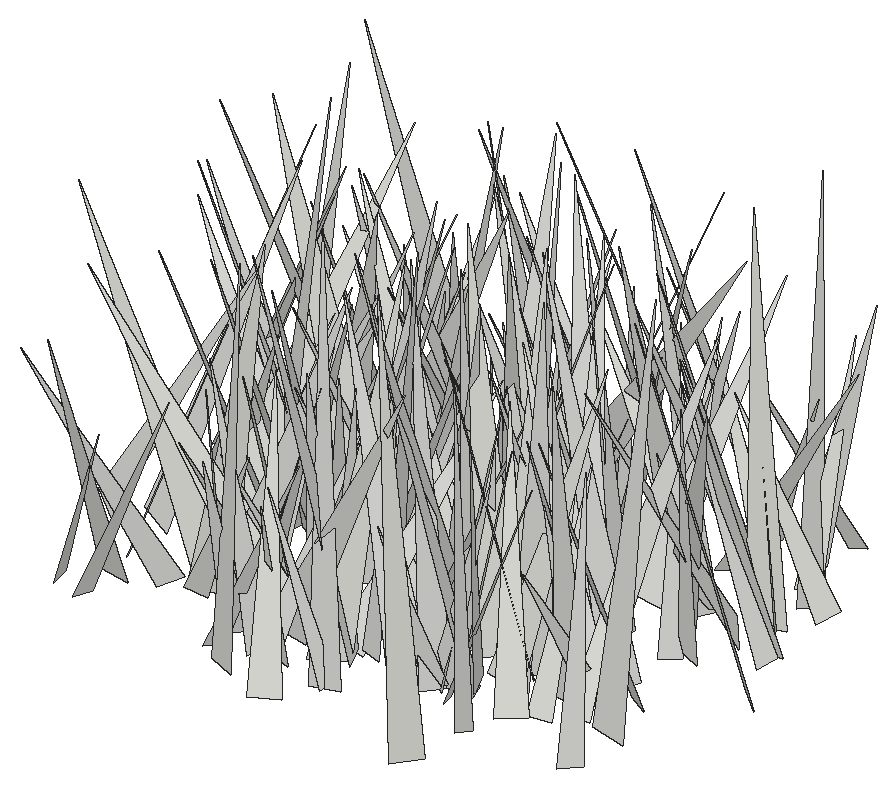
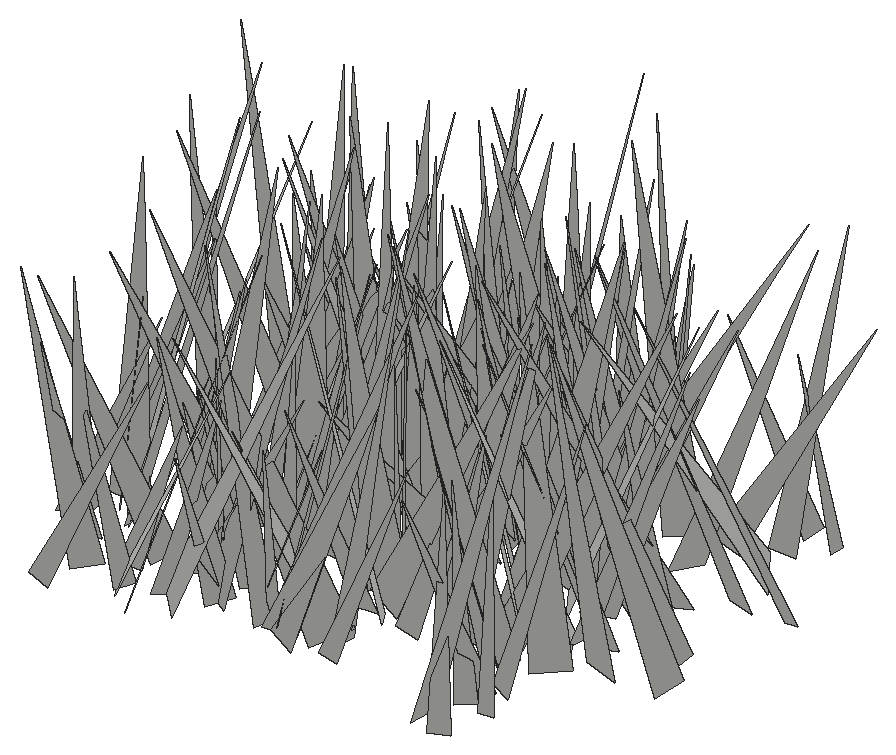
# SketchUp Ruby script. Lengths in inches.
U = 1.inch
M = Sketchup.active_model
def pt(a) = Geom::Point3d.new(a.map { |v| v * U })
def face(e, loops, mat)
  f = e.add_face(loops[0].map { |a| pt(a) })
  loops[1..].each { |l| e.add_face(l.map { |a| pt(a) }).erase! }
  f.material = f.back_material = mat if mat
  f
end
# faces: each face lists its corners as indices into pts; further lists are holes
def faces(e, pts, list, mat = nil) = list.each { |f| face(e, (f[0].is_a?(Array) ? f : [f]).map { |l| l.map { |i| pts[i] } }, mat) }
# xy, xz, yz: faces in a plane at the given z, y or x. An outline is a flat list of corners, or four numbers for a rectangle; further outlines are holes
def ring(l) = l.size == 4 ? [[l[0], l[1]], [l[2], l[1]], [l[2], l[3]], [l[0], l[3]]] : l.each_slice(2).to_a
def flat(e, list, mat, &to3) = list.each { |f| face(e, (f[0].is_a?(Array) ? f : [f]).map { |l| ring(l).map { |u, v| to3.(u, v) } }, mat) }
def xy(e, z, list, mat = nil) = flat(e, list, mat) { |x, y| [x, y, z] }
def xz(e, y, list, mat = nil) = flat(e, list, mat) { |x, z| [x, y, z] }
def yz(e, x, list, mat = nil) = flat(e, list, mat) { |y, z| [x, y, z] }
def lines(e, pts, list) = list.each { |a, b| e.add_line(pt(pts[a]), pt(pts[b])) }
# prism: a flat outline (further loops are holes) pulled along v
def prism(e, loops, v, mat = nil)
  f = face(e, loops, mat); d = Geom::Vector3d.new(v.map { |x| x * U })
  f.pushpull(f.normal.samedirection?(d) ? d.length : -d.length)
end
def box(e, o, s, mat = nil) = prism(e, [[o, [o[0] + s[0], o[1], o[2]], [o[0] + s[0], o[1] + s[1], o[2]], [o[0], o[1] + s[1], o[2]]]], [0, 0, s[2]], mat)
def at(x, y, z, deg = 0) = Geom::Transformation.translation(pt([x, y, z])) * Geom::Transformation.rotation(ORIGIN, Z_AXIS, deg.degrees)
def axes(o, x, y, z) = Geom::Transformation.new([*x, 0, *y, 0, *z, 0, *pt(o).to_a, 1])
def part(name) = M.definitions.add(name)
# library, detail: a bought-in or finely detailed component or shape, given as its bounding box
def library(name, o, s) = part(name).tap { |d| box(d.entities, o, s) }
def detail(e, o, s) = box(e.add_group.entities, o, s)
def put(e, d, t, mat = nil) = e.add_instance(d, t).tap { |i| i.material = mat if mat }
def group(e, t, mat = nil) = e.add_group.tap { |g| g.transformation = t; g.material = mat if mat }.entities
root = M.entities
c1 = part("fur_instance\#9")
p = [[0.8125,0,1.79],[0.67,-0.02,1.48],[0,-0.11,0],[0,0.11,0]]
faces(c1.entities,p,[[0,1,2,3]])
put(root,c1,axes([98,397.39,-27.1],[-0.65259,-3.58567,0.77528],[-3.62638,0.74954,0.41412],[0.55447,0.682,3.62097]))
put(root,c1,axes([89.63,398.5625,-27.1],[-0.57876,-6.04691,0.53315],[-6.05695,0.61084,0.35302],[0.40347,0.49606,6.06428]))
put(root,c1,axes([99.22,394.98,-27.1],[-1.93628,5.55,0.46539],[5.55779,1.89356,0.54185],[-0.36056,-0.61659,5.85304]))
put(root,c1,axes([96.62,395.82,-27.1],[3.17531,6.56755,2.54139],[6.79761,-3.58673,0.77578],[-1.83954,-1.91744,7.25351]))
put(root,c1,axes([95.52,398.04,-27.1],[2.55514,-3.36467,0.69917],[-3.31318,-2.64324,-0.61213],[-0.91251,0.1757,4.18031]))
put(root,c1,axes([100.41,397.04,-27.1],[-3.8674,0.14725,0.40736],[0.1724,3.88071,0.23399],[0.39736,-0.25058,3.86312]))
put(root,c1,axes([105.92,394.58,-27.1],[-8.22184,1.12863,0.67504],[0.91948,7.98903,-2.15825],[0.94024,2.05661,8.01339]))
put(root,c1,axes([88.22,397.28,-27.1],[3.62066,0.28745,0.41277],[0.34104,-3.60783,-0.479],[-0.36973,-0.51296,3.60033]))
put(root,c1,axes([95.45,396.87,-27.1],[4.11337,-1.35782,0.42666],[-1.42017,-4.00175,0.95638],[-0.09392,1.04301,4.22479]))
put(root,c1,axes([95.85,397.16,-27.1],[-3.35833,-3.2337,1.73378],[-3.57177,3.41915,-0.54142],[0.83981,1.61055,4.63056]))
put(root,c1,axes([89.6,396.83,-27.1],[4.44559,-0.41699,0.42413],[-0.48383,-4.39553,0.74982],[-0.34594,0.78895,4.4017]))
put(root,c1,axes([96.93,397.62,-27.1],[-5.40914,1.11965,1.3835],[1.23539,5.5484,0.3398],[1.28121,-0.62292,5.51334]))
put(root,c1,axes([91.48,399.41,-27.1],[0.83306,-5.07313,1.39633],[-4.3947,-1.44829,-2.63999],[-2.89363,0.73905,4.41148]))
put(root,c1,axes([103.39,399.39,-27.1],[1.75124,-3.26229,0.83742],[-3.12175,-1.92651,-0.97669],[-1.26432,0.23809,3.57148]))
put(root,c1,axes([96.93,399.07,-27.1],[2.93254,-6.52755,1.0505],[-6.19008,-2.30697,2.94501],[2.32281,2.09313,6.52193]))
put(root,c1,axes([96.53,399.75,-27.1],[-0.29394,-4.28793,0.2812],[-4.0742,0.18848,-1.38464],[-1.36614,0.36048,4.06885]))
put(root,c1,axes([96.73,400.14,-27.1],[-3.34858,-4.98605,1.16696],[-4.83329,3.53804,1.24784],[1.69169,0.23891,5.87509]))
put(root,c1,axes([99.67,399.53,-27.1],[-7.3935,-3.44968,1.78048],[-3.41196,7.60131,0.55924],[1.85173,0.23234,8.13949]))
put(root,c1,axes([96.3,399.9,-27.1],[-7.10232,2.48969,0.17848],[2.39972,6.66255,2.55443],[-0.68683,-2.46683,7.07929]))
put(root,c1,axes([92.61,399.39,-27.1],[1.69765,-3.69471,0.41656],[-3.54176,-1.46758,1.41724],[1.13153,0.9496,3.81108]))
put(root,c1,axes([100.46,396.83,-27.1],[1.13757,8.04859,1.54719],[7.76789,-1.55698,2.3882],[-2.61411,-1.12413,7.76984]))
put(root,c1,axes([97.34,397.36,-27.1],[-2.89965,3.32427,1.06428],[2.78447,3.03733,-1.90073],[2.1048,0.5615,3.98069]))
put(root,c1,axes([110.67,397.78,-27.1],[-4.9436,1.78617,0.77223],[1.56135,4.89918,-1.33648],[1.16143,1.01666,5.08364]))
put(root,c1,axes([106.16,397.46,-27.1],[-6.18556,-0.57175,1.0735],[-0.94708,5.75521,-2.39186],[0.76312,2.5082,5.73298]))
put(root,c1,axes([104.51,400.33,-27.1],[-4.3896,-2.50757,2.34029],[-2.3133,4.97071,0.98703],[2.5325,0.19407,4.95805]))
put(root,c1,axes([102.49,399.06,-27.1],[-6.29408,3.56033,1.19684],[3.6784,6.31519,0.55815],[0.76008,-1.07993,7.20971]))
put(root,c1,axes([103.33,399.73,-27.1],[0.04539,-4.24616,1.86431],[-4.44886,0.48634,1.21602],[1.30888,1.80033,4.06857]))
put(root,c1,axes([95.48,399.4,-27.1],[5.08569,0.11573,0.95874],[0.07501,-5.17107,0.22632],[-0.96278,0.20845,5.08197]))
put(root,c1,axes([93.01,399.72,-27.1],[-2.73382,6.12597,3.74599],[6.6709,3.64992,-1.10045],[2.6569,-2.86083,6.61742]))
put(root,c1,axes([96.35,401.17,-27.1],[-3.41179,-1.77285,0.16017],[-1.67154,3.30984,1.02951],[0.61205,-0.84317,3.70451]))
put(root,c1,axes([96.98,401.18,-27.1],[3.24454,-4.71501,1.03025],[-4.7617,-3.32972,-0.24278],[-0.78672,0.70811,5.71834]))
put(root,c1,axes([104.32,398.85,-27.1],[3.89284,1.77366,0.49192],[1.64576,-3.86945,0.92782],[-0.82421,0.65077,4.17603]))
put(root,c1,axes([104.79,399.78,-27.1],[-7.44301,-3.63877,0.95843],[-3.76282,7.20814,-1.85509],[0.01898,2.08796,8.0745]))
put(root,c1,axes([98.05,400.78,-27.1],[4.42383,-2.92058,1.2942],[-2.99041,-4.56361,-0.07677],[-1.12348,0.64702,5.30039]))
put(root,c1,axes([100.23,399.66,-27.1],[-1.46329,-3.87448,2.4887],[-4.52721,1.6881,-0.03379],[0.84239,2.34204,4.14146]))
put(root,c1,axes([108.59,402.04,-27.1],[2.63611,-2.6678,0.56163],[-2.26437,-2.5776,-1.61563],[-1.51829,-0.78771,3.38467]))
put(root,c1,axes([99.3,398.49,-27.1],[-5.55671,4.70477,2.20019],[4.40361,5.97611,-1.65743],[2.7539,-0.06297,7.08977]))
put(root,c1,axes([103.92,400.03,-27.1],[4.05853,2.67005,1.15678],[2.78357,-4.14094,-0.20805],[-0.84796,-0.81387,4.85361]))
put(root,c1,axes([107.83,401.4,-27.1],[0.14601,-6.62439,2.10053],[-6.94709,-0.08453,0.21629],[0.18059,2.1039,6.62247]))
put(root,c1,axes([106.84,399.27,-27.1],[-4.29612,3.71614,0.38084],[3.69784,4.31285,-0.36964],[0.52979,0.03157,5.66831]))
put(root,c1,axes([101.72,403.07,-27.1],[-1.16201,-7.65185,1.0654],[-7.72512,1.16361,-0.06847],[0.09162,1.06366,7.73928]))
put(root,c1,axes([91.57,401.52,-27.1],[-7.37091,1.53228,0.84327],[1.65266,7.29739,1.18581],[0.57246,-1.33774,7.43452]))
put(root,c1,axes([105.21,402.41,-27.1],[-4.80805,-4.95386,1.3489],[-5.02147,4.92244,0.17909],[1.0701,0.84054,6.90116]))
put(root,c1,axes([107.86,401.81,-27.1],[1.52237,-3.55739,1.37163],[-3.65271,-1.78416,-0.57315],[-1.09275,1.00785,3.82677]))
put(root,c1,axes([103.53,399.18,-27.1],[-7.58228,1.17889,0.51367],[1.00041,7.33787,-2.07353],[0.80796,1.97752,7.38791]))
put(root,c1,axes([103.68,399.24,-27.1],[3.73526,4.02595,0.93613],[3.5763,-3.78049,1.98866],[-2.07237,0.73241,5.11915]))
put(root,c1,axes([109.67,402.8125,-27.1],[-3.13069,-4.74867,0.6646],[-4.79451,3.11096,-0.35688],[0.06511,0.75154,5.67659]))
put(root,c1,axes([107.67,399.79,-27.1],[-0.4926,4.67354,0.05511],[4.67276,0.49124,0.10792],[-0.10156,-0.0661,4.69819]))
put(root,c1,axes([110.29,400.34,-27.1],[2.12447,7.8086,2.15105],[8.03257,-2.31646,0.47574],[-1.03873,-1.94278,8.07844]))
put(root,c1,axes([99.2,399.68,-27.1],[-0.72981,5.66267,0.18679],[5.27184,0.7477,-2.06932],[2.0757,0.09199,5.32132]))
put(root,c1,axes([95.5,403.39,-27.1],[-0.07367,-4.26522,0.50041],[-4.16979,0.19077,1.01214],[1.02732,0.46845,4.14405]))
put(root,c1,axes([105.45,402.17,-27.1],[1.282,-6.99581,3.06835],[-7.6361,-1.26107,0.31524],[-0.21483,3.07701,7.10532]))
put(root,c1,axes([105.08,401.09,-27.1],[0.03903,6.40601,1.64221],[6.43648,0.34027,-1.48032],[1.51842,-1.60705,6.23275]))
put(root,c1,axes([98.98,402.36,-27.1],[7.15031,1.42356,2.57616],[1.59453,-7.56218,-0.24693],[-2.47399,-0.75958,7.28646]))
put(root,c1,axes([108.72,400.625,-27.1],[-1.96871,3.37657,0.07437],[3.27614,1.93014,-0.90775],[0.82077,0.39482,3.80171]))
put(root,c1,axes([101.26,400.78,-27.1],[4.64309,0.99306,0.50279],[0.80416,-4.48393,1.43003],[-0.7696,1.30595,4.52764]))
put(root,c1,axes([100.41,402.65,-27.1],[-3.73947,1.85603,0.44676],[1.90802,3.6015,1.00834],[-0.06253,-1.10111,4.05114]))
put(root,c1,axes([96.15,403.49,-27.1],[4.14097,0.37336,0.37849],[0.46882,-3.96604,-1.21698],[-0.25072,-1.24957,3.97567]))
put(root,c1,axes([106.59,404.04,-27.1],[-1.84979,-4.95748,0.73449],[-4.97918,1.90688,0.3307],[0.56907,0.57009,5.281]))
put(root,c1,axes([95.66,403.45,-27.1],[0.8315,-3.67241,0.7269],[-3.73531,-0.86356,-0.09004],[-0.24991,0.6885,3.76429]))
put(root,c1,axes([95.33,404.04,-27.1],[0.2797,-5.08952,0.70223],[-5.01624,-0.11848,1.13926],[1.11073,0.74654,4.96825]))
put(root,c1,axes([108.11,402.18,-27.1],[-4.76226,4.46867,0.77555],[4.53262,4.64929,1.04363],[-0.16086,-1.29026,6.44663]))
put(root,c1,axes([93.45,403.39,-27.1],[-3.66042,-4.84933,0.70173],[-4.78346,3.34689,-1.82316],[-1.06154,1.63996,5.79575]))
put(root,c1,axes([102.76,402.32,-27.1],[-6.8831,0.44539,2.18741],[0.27023,7.20464,-0.61666],[2.21588,0.50489,6.86987]))
put(root,c1,axes([92.375,402.62,-27.1],[1.25839,-5.65908,2.69216],[-6.0262,-0.33916,2.10388],[1.71982,2.95233,5.40207]))
put(root,c1,axes([103.74,402.46,-27.1],[-6.05615,5.17907,2.30301],[5.46239,6.23254,0.34836],[1.51293,-1.77094,7.96105]))
put(root,c1,axes([102.32,403.3,-27.1],[2.05705,-3.40779,1.21765],[-3.60141,-2.06493,0.30505],[-0.3543,1.20424,3.9688]))
put(root,c1,axes([92.71,405.33,-27.1],[-2.90954,-6.16313,0.64564],[-6.10361,2.97343,0.8781],[1.07095,0.20243,6.75859]))
put(root,c1,axes([86.18,402.37,-27.1],[3.46284,5.45761,0.55951],[5.19477,-3.049,-2.40992],[1.76435,-1.73432,5.99742]))
put(root,c1,axes([98.26,405.3,-27.1],[-5.70608,-2.81682,0.48614],[-2.67601,5.6456,1.30244],[1.0049,-0.96065,6.22877]))
put(root,c1,axes([96.38,404.87,-27.1],[-4.22859,-0.79072,0.99748],[-0.41595,4.12901,1.5098],[1.20299,-1.35177,4.02824]))
put(root,c1,axes([94.06,405.22,-27.1],[-1.823,-5.96341,0.88128],[-5.94354,1.93183,0.77754],[1.00658,0.60664,6.18716]))
put(root,c1,axes([100.49,404.15,-27.1],[6.63287,-1.89646,1.66739],[-1.83678,-6.83922,-0.47211],[-1.73291,-0.0097,6.88248]))
put(root,c1,axes([105.97,400.49,-27.1],[-6.32088,1.55628,0.92222],[1.03646,5.86264,-2.78949],[1.48264,2.53644,5.88169]))
put(root,c1,axes([107.03,403.59,-27.1],[-1.92463,-5.23066,1.71698],[-5.26178,1.21283,-2.20335],[-1.6191,2.27625,5.1195]))
put(root,c1,axes([104.8125,402.0625,-27.1],[-1.18605,7.62635,1.82441],[7.84154,1.15487,0.27022],[0.00582,-1.84431,7.7133]))
put(root,c1,axes([93.46,402.88,-27.1],[0.89706,4.01856,0.51185],[4.05094,-0.89322,-0.08685],[-0.02607,-0.51851,4.11655]))
put(root,c1,axes([92.5,405.0625,-27.1],[6.03259,-1.06555,0.38284],[-1.02373,-6.01977,-0.62323],[-0.48366,-0.54868,6.09418]))
put(root,c1,axes([102.65,402.875,-27.1],[-4.5808,2.50643,0.71678],[2.42315,4.62824,-0.69815],[0.96142,0.27723,5.1748]))
put(root,c1,axes([88.34,402.5,-27.1],[3.15625,6.97995,0.87784],[7.00121,-3.02246,-1.14023],[0.68808,-1.26383,7.57506]))
put(root,c1,axes([112.61,405.41,-27.1],[-5.20648,-5.71637,1.32602],[-5.85189,5.18966,-0.6046],[0.43665,1.3904,7.70836]))
put(root,c1,axes([108.56,403.31,-27.1],[-7.87651,1.28049,0.44694],[1.23259,7.85729,-0.78901],[0.56579,0.70864,7.94081]))
put(root,c1,axes([89.11,399.98,-27.1],[6.66219,5.05954,0.23915],[4.47229,-6.06129,3.64695],[-2.37798,2.77537,7.52884]))
put(root,c1,axes([98.6875,404.67,-27.1],[-2.55012,3.64542,1.48438],[3.93085,2.44958,0.73729],[0.20222,-1.64502,4.38733]))
put(root,c1,axes([97.36,403.51,-27.1],[5.64038,0.84844,0.8162],[0.68974,-5.61874,1.07421],[-0.95409,0.95384,5.60177]))
put(root,c1,axes([96.61,403.33,-27.1],[6.53232,-2.04401,3.08815],[-2.89411,-6.72439,1.67109],[-2.31057,2.64395,6.63752]))
put(root,c1,axes([103.83,406.2,-27.1],[-3.87501,-4.05549,0.17386],[-4.05477,3.85598,-0.42797],[-0.18982,0.42113,5.59281]))
put(root,c1,axes([95.58,404.09,-27.1],[6.99973,1.86447,1.44835],[1.77883,-7.14461,0.6004],[-1.55233,0.22015,7.21886]))
put(root,c1,axes([89,405.9,-27.1],[3.52002,-2.83902,0.00242],[-2.82378,-3.50072,0.47096],[0.29379,0.3681,4.49764]))
put(root,c1,axes([106.98,403.66,-27.1],[0.16958,6.97336,1.46095],[6.91324,0.19239,-1.72074],[1.72314,-1.45812,6.75984]))
put(root,c1,axes([97.67,404.49,-27.1],[4.97353,-2.18793,2.98402],[-2.79783,-5.49524,0.634],[-2.42149,1.85546,5.39639]))
put(root,c1,axes([103.84,404.8125,-27.1],[-5.54027,1.19429,0.93196],[1.15956,5.61711,-0.30487],[0.97482,0.10593,5.65933]))
put(root,c1,axes([109.23,408.98,-27.1],[-5.37416,-4.85351,0.14678],[-4.51514,5.07548,2.5125],[1.7865,-1.77274,6.79157]))
put(root,c1,axes([93.1,406.25,-27.1],[-5.86461,-3.9483,0.52207],[-3.9663,5.70596,-1.40208],[-0.36068,1.452,6.92942]))
put(root,c1,axes([106.74,408.79,-27.1],[-0.05965,-7.49908,0.31223],[-6.76708,0.1888,3.24163],[3.24657,0.25574,6.76251]))
put(root,c1,axes([101.02,404.87,-27.1],[6.96857,2.87265,0.80723],[2.85827,-7.01507,0.2896],[-0.85676,-0.03815,7.53188]))
put(root,c1,axes([103.38,407.47,-27.1],[-6.6748,0.96554,1.83268],[1.43583,6.61336,1.7452],[1.49311,-2.0433,6.51456]))
put(root,c1,axes([91.78,404.85,-27.1],[4.31651,6.80061,2.35568],[7.01576,-4.58865,0.3914],[-1.60519,-1.76799,8.04533]))
put(root,c1,axes([108.96,406.5,-27.1],[-1.48378,-4.80354,1.85374],[-5.06695,1.70492,0.36217],[0.91449,1.65264,5.01442]))
put(root,c1,axes([99.99,408.0625,-27.1],[7.80174,-0.94154,1.76979],[-0.49694,-7.7978,-1.95786],[-1.94209,-1.78708,7.61055]))
put(root,c1,axes([94.63,405.85,-27.1],[5.61379,-0.0924,1.25595],[-0.17391,-5.73971,0.3551],[-1.24727,0.38445,5.60331]))
put(root,c1,axes([95.93,405.61,-27.1],[-2.4957,-1.61977,2.11338],[-2.18018,2.90599,-0.34732],[1.52869,1.50005,2.95492]))
put(root,c1,axes([91.89,406.08,-27.1],[-4.33384,4.15795,0.46311],[4.09626,4.08164,1.68703],[-0.85069,-1.52868,5.76409]))
put(root,c1,axes([97.25,405.2,-27.1],[1.39427,3.92432,0.17719],[3.92808,-1.39069,-0.10895],[0.04345,-0.20342,4.16322]))
put(root,c1,axes([99.05,405.45,-27.1],[-3.57557,6.64036,0.56629],[6.42877,3.26724,2.27945],[-1.75672,-1.55901,7.1891]))
put(root,c1,axes([105.2,405.3,-27.1],[-2.95766,6.66869,1.17233],[6.76114,2.97762,0.11972],[0.36439,-1.12067,7.29416]))
put(root,c1,axes([90.14,403.95,-27.1],[0.04279,8.23701,0.26485],[7.98617,0.02394,-2.03491],[2.0346,-0.26721,7.98181]))
put(root,c1,axes([94.18,407.33,-27.1],[-5.61004,5.72169,2.32507],[6.16954,5.3361,1.75473],[0.28367,-2.89906,7.81865]))
put(root,c1,axes([104.67,407.73,-27.1],[-5.00716,-3.11226,0.75462],[-3.18598,4.98296,-0.58898],[0.32424,0.90067,5.86608]))
put(root,c1,axes([106.28,406.3,-27.1],[-7.03444,-1.19576,1.59787],[-1.52444,6.99776,-1.47438],[1.28808,1.75153,6.98136]))
put(root,c1,axes([91.1875,407.82,-27.1],[-6.42244,0.41118,0.57395],[0.45958,6.42194,0.54196],[0.53597,-0.57954,6.41273]))
put(root,c1,axes([100.18,404.72,-27.1],[-3.33289,3.23483,0.32122],[2.5841,2.91556,-2.549],[1.97223,1.64647,3.88264]))
put(root,c1,axes([111.12,408.46,-27.1],[-1.48365,-5.76059,1.44193],[-5.8771,1.21156,-1.20691],[-0.85046,1.67706,5.82486]))
put(root,c1,axes([98.6875,408.46,-27.1],[3.47548,2.68418,2.07766],[3.24177,-3.50628,-0.89294],[-1.00618,-2.02524,4.29959]))
put(root,c1,axes([89.91,407.73,-27.1],[2.31497,4.33574,1.17317],[4.28428,-1.73503,-2.04175],[1.34907,-1.93005,4.47091]))
put(root,c1,axes([111.43,407.99,-27.1],[-5.40823,0.65228,0.52882],[0.69912,5.40686,0.48075],[0.46513,-0.5426,5.42617]))
put(root,c1,axes([99.375,407.87,-27.1],[-2.0645,-2.99831,1.70133],[-3.28642,2.31061,0.08412],[1.04107,1.34824,3.63936]))
put(root,c1,axes([108.54,406.05,-27.1],[-4.64664,1.60589,0.29185],[1.45378,4.47236,-1.46283],[0.74202,1.29401,4.69365]))
put(root,c1,axes([87.43,406.98,-27.1],[6.02676,-0.13267,0.65935],[-0.25057,-5.95995,1.09109],[-0.62414,1.1116,5.92866]))
put(root,c1,axes([107.24,409.38,-27.1],[2.57242,-3.23839,0.522],[-3.12857,-2.6216,-0.84629],[-0.98573,-0.13048,4.04824]))
put(root,c1,axes([108.75,411.08,-27.1],[-6.83559,-3.49227,1.59422],[-2.83471,6.78714,2.71329],[2.5888,-1.7893,7.18049]))
put(root,c1,axes([103.24,408.25,-27.1],[-3.28307,2.60382,1.30489],[2.8552,3.26547,0.66758],[0.57484,-1.34832,4.13676]))
put(root,c1,axes([93.46,408.93,-27.1],[-3.35024,-7.10363,1.41562],[-6.97339,2.74138,-2.74705],[-1.95891,2.39017,7.35795]))
put(root,c1,axes([97.37,408.04,-27.1],[-4.10469,4.34568,0.4298],[4.19686,3.76273,2.03626],[-1.20665,-1.6956,5.62024]))
put(root,c1,axes([90.53,407.73,-27.1],[3.62784,4.7769,0.79864],[4.78599,-3.38301,-1.50576],[0.74217,-1.53438,5.80626]))
put(root,c1,axes([93.03,408.84,-27.1],[5.29628,3.42643,1.15131],[3.61426,-4.98862,-1.7797],[0.0553,-2.11891,6.05175]))
put(root,c1,axes([104.26,406.95,-27.1],[-3.06885,7.2619,1.47031],[7.40414,2.94663,0.90053],[-0.27521,-1.70206,7.83212]))
put(root,c1,axes([90.62,410.27,-27.1],[3.94338,-5.9757,0.15667],[-5.94055,-3.89659,0.90015],[0.66588,0.62564,7.10275]))
put(root,c1,axes([103.9375,408.34,-27.1],[-4.03311,-0.04964,1.55556],[-0.10181,4.31995,-0.1261],[1.55302,0.15428,4.03144]))
put(root,c1,axes([97.29,406.27,-27.1],[-7.34355,0.30763,3.29021],[-0.75169,7.65215,-2.39318],[3.21793,2.48952,6.94946]))
put(root,c1,axes([109.02,410.93,-27.1],[-5.87389,-5.06073,1.31002],[-4.91563,6.01764,1.20596],[1.77871,-0.08191,7.65893]))
put(root,c1,axes([86.6,408.65,-27.1],[6.73911,-0.51973,0.37006],[-0.5475,-6.72675,0.52311],[-0.32757,0.55072,6.73884]))
put(root,c1,axes([96,409.22,-27.1],[1.13242,-3.28388,1.61058],[-3.44754,-1.52145,-0.67814],[-1.2216,1.24962,3.40681]))
put(root,c1,axes([101.37,408.59,-27.1],[-2.35431,6.5098,1.98677],[6.74258,1.94391,1.62058],[-0.92858,-2.38982,6.73008]))
put(root,c1,axes([96.31,411.22,-27.1],[-1.09873,-5.30096,0.04279],[-5.29764,1.09638,-0.20521],[-0.19227,0.08352,5.40974]))
put(root,c1,axes([91.31,408.14,-27.1],[5.4364,3.24485,0.19999],[3.25087,-5.4295,-0.27539],[-0.03035,-0.33899,6.32516]))
put(root,c1,axes([94.55,410.31,-27.1],[0.42808,-6.23217,1.75974],[-6.34467,-0.7568,-1.13683],[-1.29687,1.64535,6.14254]))
put(root,c1,axes([98.25,410.1,-27.1],[-2.1287,-6.56011,1.58213],[-6.38568,1.42177,-2.69649],[-2.18201,2.23898,6.34786]))
put(root,c1,axes([104.99,411.33,-27.1],[0.47812,-7.3143,1.47747],[-7.45136,-0.54714,-0.29732],[-0.39895,1.45332,7.32388]))
put(root,c1,axes([92.34,410.92,-27.1],[1.4912,-7.63112,1.5604],[-7.07021,-0.65953,3.53123],[3.26816,2.05513,6.92734]))
put(root,c1,axes([100.98,407.57,-27.1],[3.07038,6.62387,1.59445],[6.28566,-3.42873,2.13997],[-2.62838,-0.46188,6.98022]))
put(root,c1,axes([97.57,410.99,-27.1],[6.19787,3.91116,1.13836],[4.069,-5.84754,-2.06304],[0.19042,-2.34857,7.0324]))
put(root,c1,axes([99.47,410.57,-27.1],[-5.53788,-5.2946,2.37412],[-5.70348,5.57065,-0.88067],[1.06751,2.29618,7.61087]))
put(root,c1,axes([89.26,409.18,-27.1],[1.99412,7.08431,1.8343],[7.27705,-2.12036,0.27805],[-0.77249,-1.68678,7.35436]))
put(root,c1,axes([109.78,409.88,-27.1],[-0.81741,7.52572,2.31704],[7.8363,0.54876,0.98214],[-0.77303,-2.39493,7.506]))
put(root,c1,axes([98.56,409.37,-27.1],[-2.23719,7.0676,1.63885],[7.20712,2.3619,-0.34736],[0.83319,-1.45336,7.40509]))
put(root,c1,axes([105.26,408.73,-27.1],[-1.51128,6.4389,0.97646],[6.11666,1.74753,-2.05657],[2.23592,-0.42848,6.28601]))
put(root,c1,axes([110.18,409.91,-27.1],[-4.46035,-2.40279,1.6408],[-2.85913,4.17643,-1.65628],[0.53948,2.26814,4.788]))
put(root,c1,axes([91.15,412.45,-27.1],[-2.16973,-4.86696,0.63571],[-4.9077,2.16207,-0.19771],[0.07681,0.6613,5.32503]))
put(root,c1,axes([107.52,409.27,-27.1],[-7.36083,-0.13148,0.37404],[-0.23398,7.05478,-2.12469],[0.32007,2.13349,7.04874]))
put(root,c1,axes([105.9375,409.52,-27.1],[-2.69846,2.82224,0.09608],[2.72603,2.63813,-0.93001],[0.73688,0.57546,3.79233]))
put(root,c1,axes([111.05,411.75,-27.1],[-4.33776,1.46199,0.55548],[1.55819,4.18055,1.16497],[0.13425,-1.28363,4.42678]))
put(root,c1,axes([100.25,413.4,-27.1],[-5.41835,-3.58553,1.38238],[-3.2455,5.54933,1.6725],[2.0576,-0.68883,6.27832]))
put(root,c1,axes([102.42,411.1875,-27.1],[-3.43885,-1.25141,0.28396],[-1.28081,3.29756,-0.97876],[-0.07859,1.01608,3.52615]))
put(root,c1,axes([91.88,411.56,-27.1],[3.27603,2.91205,0.73309],[2.99826,-3.11162,-1.03833],[0.1671,-1.26001,4.25844]))
put(root,c1,axes([102.64,412.15,-27.1],[0.8957,-3.44027,0.95903],[-3.38159,-0.49886,1.36875],[1.14894,1.21373,3.28089]))
put(root,c1,axes([103.05,413.53,-27.1],[-3.74984,-6.28849,1.24601],[-6.40364,3.74219,-0.38514],[0.30173,1.26879,7.3115]))
put(root,c1,axes([104.47,412.28,-27.1],[-4.30239,2.31555,0.00735],[2.25428,4.18495,1.12996],[-0.52922,-0.99839,4.75348]))
put(root,c1,axes([98.13,413.15,-27.1],[4.31656,-7.06636,0.27005],[-6.24466,-3.6606,4.0303],[3.31821,2.3034,7.23345]))
put(root,c1,axes([106.26,412.25,-27.1],[4.90095,-2.69617,0.00541],[-2.57457,-4.67657,1.67032],[0.80058,1.46597,5.33842]))
put(root,c1,axes([103.5,412.54,-27.1],[2.79577,3.11606,1.7882],[3.42019,-3.00212,-0.11591],[-1.09992,-1.41467,4.18482]))
put(root,c1,axes([100.33,411.18,-27.1],[3.37937,2.22818,0.23171],[2.15143,-3.34494,0.78826],[-0.62436,0.53406,3.97033]))
put(root,c1,axes([98.47,410.83,-27.1],[-0.0626,5.05917,0.30688],[5.04763,0.09003,-0.45456],[0.45914,-0.29998,5.03909]))
put(root,c1,axes([100.6,413.76,-27.1],[6.84395,0.46131,0.76105],[0.6015,-6.74756,-1.31919],[-0.65589,-1.3745,6.73144]))
put(root,c1,axes([97.61,413.26,-27.1],[5.36084,-0.19835,3.29768],[0.06393,-6.27827,-0.48156],[-3.30302,-0.44345,5.34285]))
put(root,c1,axes([91.51,413.92,-27.1],[1.83451,-3.56347,0.05806],[-3.52397,-1.80394,0.62811],[0.53227,0.33851,3.95843]))
put(root,c1,axes([90.5,414.0625,-27.1],[-0.97115,-4.17934,0.95629],[-4.09852,1.19278,1.05068],[1.25838,0.65947,4.16006]))
put(root,c1,axes([99.59,414.33,-27.1],[-2.75065,-6.97463,1.22589],[-6.99898,2.47729,-1.60986],[-1.07823,1.71227,7.32256]))
put(root,c1,axes([97.34,414.36,-27.1],[-0.13278,-3.81265,0.23397],[-3.74221,0.08288,-0.77308],[-0.76609,0.25594,3.73581]))
put(root,c1,axes([102.79,413.57,-27.1],[4.10289,-2.86128,0.97197],[-3.01034,-4.01302,0.89377],[-0.2636,1.29386,4.92156]))
put(root,c1,axes([104.27,414.61,-27.1],[-5.74525,-5.95088,0.61636],[-5.93253,5.55629,-1.65334],[-0.77329,1.58601,8.10478]))
put(root,c1,axes([104.72,414.4,-27.1],[-3.60372,1.36671,1.25031],[1.68423,3.55609,0.96723],[0.77106,-1.37995,3.73084]))
put(root,c1,axes([99.84,413.96,-27.1],[-3.57331,4.48467,0.98446],[4.4978,3.16833,1.89248],[-0.92266,-1.92337,5.41289]))
put(root,c1,axes([106.88,413.51,-27.1],[-1.92431,3.57441,0.40694],[3.46774,1.72017,1.28872],[-0.95749,-0.95373,3.84949]))
put(root,c1,axes([109.36,412.72,-27.1],[-0.62067,4.74172,0.56344],[4.77083,0.63973,-0.12835],[0.20124,-0.5417,4.78044]))
put(root,c1,axes([100.51,413.42,-27.1],[1.055,3.81063,1.04337],[3.83467,-1.24762,0.6792],[-0.95124,-0.80317,3.89521]))
put(root,c1,axes([99.24,412.1,-27.1],[5.73522,3.47371,0.17785],[3.39582,-5.66618,1.16354],[-0.75282,0.90483,6.60345]))
put(root,c1,axes([91.6,412.8,-27.1],[-0.33332,4.6985,0.41104],[4.65173,0.39553,-0.74898],[0.77866,-0.35159,4.65038]))
put(root,c1,axes([106.1,414.79,-27.1],[3.40491,-1.73217,0.1961],[-1.74293,-3.39081,0.31125],[-0.03288,0.3664,3.80749]))
put(root,c1,axes([105.3,415.5,-27.1],[-6.81995,-3.62088,0.84533],[-3.65528,6.85252,-0.13797],[0.68141,0.51893,7.72033]))
put(root,c1,axes([106.34,414.87,-27.1],[-4.80301,-2.64529,0.12183],[-2.62964,4.73476,-0.865],[-0.31202,0.81591,5.41463]))
put(root,c1,axes([92.15,415.375,-27.1],[-7.83608,-0.63477,1.59162],[-0.4911,7.96997,0.76075],[1.64165,-0.64574,7.82485]))
put(root,c1,axes([108,414.48,-27.1],[-1.7832,4.7887,2.83203],[5.02838,2.65983,-1.33139],[2.38064,-2.03113,4.93345]))
put(root,c1,axes([110.11,411.95,-27.1],[-7.67594,0.43258,1.18162],[-0.05572,7.18028,-2.99063],[1.25708,2.9597,7.0826]))
put(root,c1,axes([103.39,413.21,-27.1],[0.25291,3.93977,0.05992],[3.89833,-0.25892,0.57035],[-0.57304,-0.02262,3.90646]))
put(root,c1,axes([108.74,416.31,-27.1],[-0.19761,-4.29399,0.26182],[-4.09062,0.10641,-1.34218],[-1.33181,0.31028,4.08362]))
put(root,c1,axes([90.93,416.17,-27.1],[0.8236,-4.35079,0.44599],[-4.32851,-0.74586,0.71716],[0.62636,0.56649,4.3696]))
